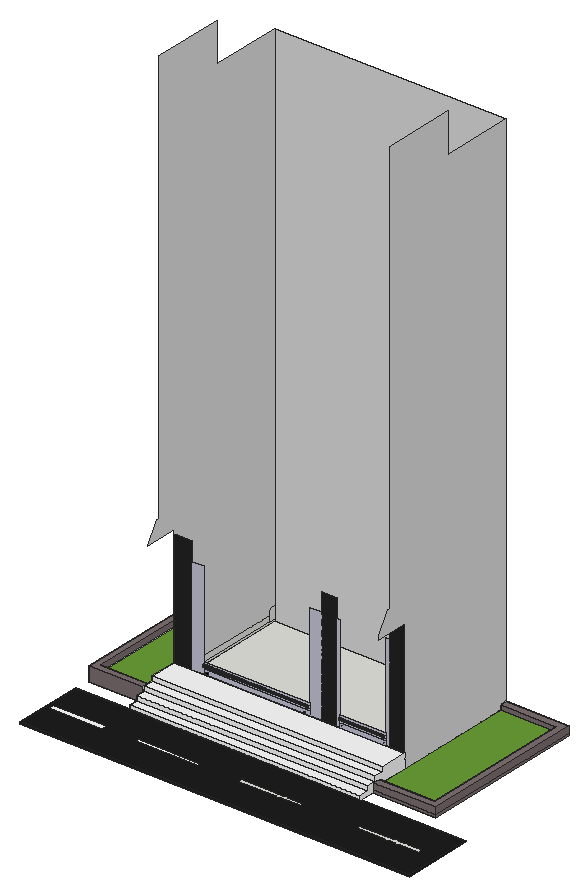
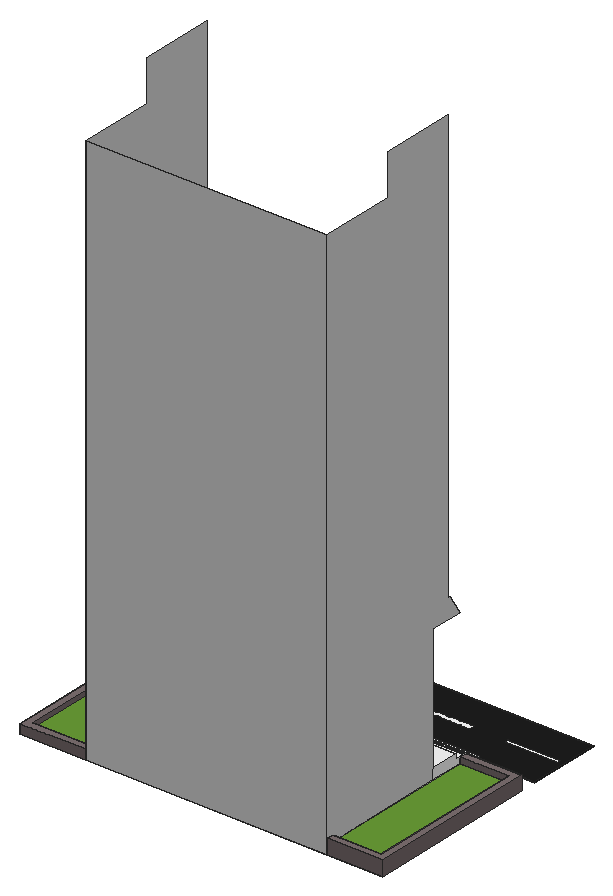
# SketchUp Ruby script. Lengths in millimetres.
U = 1.mm
M = Sketchup.active_model
def pt(a) = Geom::Point3d.new(a.map { |v| v * U })
def face(e, loops, mat)
  f = e.add_face(loops[0].map { |a| pt(a) })
  loops[1..].each { |l| e.add_face(l.map { |a| pt(a) }).erase! }
  f.material = f.back_material = mat if mat
  f
end
# faces: each face lists its corners as indices into pts; further lists are holes
def faces(e, pts, list, mat = nil) = list.each { |f| face(e, (f[0].is_a?(Array) ? f : [f]).map { |l| l.map { |i| pts[i] } }, mat) }
# xy, xz, yz: faces in a plane at the given z, y or x. An outline is a flat list of corners, or four numbers for a rectangle; further outlines are holes
def ring(l) = l.size == 4 ? [[l[0], l[1]], [l[2], l[1]], [l[2], l[3]], [l[0], l[3]]] : l.each_slice(2).to_a
def flat(e, list, mat, &to3) = list.each { |f| face(e, (f[0].is_a?(Array) ? f : [f]).map { |l| ring(l).map { |u, v| to3.(u, v) } }, mat) }
def xy(e, z, list, mat = nil) = flat(e, list, mat) { |x, y| [x, y, z] }
def xz(e, y, list, mat = nil) = flat(e, list, mat) { |x, z| [x, y, z] }
def yz(e, x, list, mat = nil) = flat(e, list, mat) { |y, z| [x, y, z] }
def lines(e, pts, list) = list.each { |a, b| e.add_line(pt(pts[a]), pt(pts[b])) }
# prism: a flat outline (further loops are holes) pulled along v
def prism(e, loops, v, mat = nil)
  f = face(e, loops, mat); d = Geom::Vector3d.new(v.map { |x| x * U })
  f.pushpull(f.normal.samedirection?(d) ? d.length : -d.length)
end
def box(e, o, s, mat = nil) = prism(e, [[o, [o[0] + s[0], o[1], o[2]], [o[0] + s[0], o[1] + s[1], o[2]], [o[0], o[1] + s[1], o[2]]]], [0, 0, s[2]], mat)
def at(x, y, z, deg = 0) = Geom::Transformation.translation(pt([x, y, z])) * Geom::Transformation.rotation(ORIGIN, Z_AXIS, deg.degrees)
def axes(o, x, y, z) = Geom::Transformation.new([*x, 0, *y, 0, *z, 0, *pt(o).to_a, 1])
def part(name) = M.definitions.add(name)
# library, detail: a bought-in or finely detailed component or shape, given as its bounding box
def library(name, o, s) = part(name).tap { |d| box(d.entities, o, s) }
def detail(e, o, s) = box(e.add_group.entities, o, s)
def put(e, d, t, mat = nil) = e.add_instance(d, t).tap { |i| i.material = mat if mat }
def group(e, t, mat = nil) = e.add_group.tap { |g| g.transformation = t; g.material = mat if mat }.entities
root = M.entities
M.materials.add("[0116_Lavender]").color = [197, 197, 214]
M.materials.add("[0128_White]1").color = [255, 255, 255]
M.materials.add("[0130_Gainsboro]").color = [220, 220, 220]
M.materials.add("[0136_Charcoal]").color = [35, 35, 35]
M.materials.add("[0137_Black]").color = [0, 0, 0]
M.materials.add("[Asphalt Stamped Brick]").color = [124, 111, 112]
M.materials.add("[Blacktop New]").color = [30, 30, 30]
M.materials.add("[Carrera Marble]").color = [252, 252, 252]
M.materials.add("[Grass Dark Green]").color = [106, 157, 55]
xy(root,-136.5,[[7076.1,9232.9,37556.1,16548.1],[0,11366.5,7076.1,33312.1],[37556.1,11366.5,45838.4,33312.1],[7076.1,16548.1,37556.1,33312.1]])
xy(root,-136.5,[[0,0,51467,9232.9]],"[Blacktop New]")
xy(root,15.9,[[25341.5,4311.6,33627.1,4921.2],[40973.6,4311.6,49259.3,4921.2]])
xy(root,15.9,[[553.8,4311.6,7431.8,4921.2],[11711.2,4311.6,19996.9,4921.2]],"[0128_White]1")
xy(root,15.9,[[[0,0,51467,9232.9],[40973.6,4311.6,49259.3,4921.2],[25341.5,4311.6,33627.1,4921.2],[11711.2,4311.6,19996.9,4921.2],[553.8,4311.6,7431.8,4921.2]]],"[Blacktop New]")
xy(root,168.3,[[914.4,12280.9,7076.1,32397.7]])
xy(root,473.1,[[7076.1,9232.9,37556.1,10452.1]],"[Carrera Marble]")
xy(root,473.1,[[37556.1,12280.9,44924,32397.7]],"[Grass Dark Green]")
xy(root,930.3,[[914.4,12280.9,7076.1,32397.7]],"[Grass Dark Green]")
xy(root,1082.7,[[37556.1,11366.5,45838.4,11366.5,45838.4,33312.1,37556.1,33312.1,37556.1,32397.7,44924,32397.7,44924,12280.9,37556.1,12280.9]],"[Asphalt Stamped Brick]")
xy(root,1082.7,[[7076.1,10452.1,37556.1,11671.3]],"[Carrera Marble]")
xy(root,1692.3,[[0,11366.5,7076.1,11366.5,7076.1,12280.9,914.4,12280.9,914.4,32397.7,7076.1,32397.7,7076.1,33312.1,0,33312.1]],"[Asphalt Stamped Brick]")
xy(root,1692.3,[[7076.1,11671.3,37556.1,12890.5]],"[Carrera Marble]")
xy(root,2301.9,[[7076.1,12890.5,37556.1,16548.1]],"[Carrera Marble]")
xz(root,0,[[0,-136.5,51467,15.9]],"[Blacktop New]")
xz(root,9232.9,[[0,-136.5,7076.1,15.9],[37556.1,-136.5,51467,15.9]],"[Blacktop New]")
xz(root,9232.9,[[7076.1,-136.5,37556.1,15.9],[7076.1,15.9,37556.1,473.1]],"[Carrera Marble]")
xz(root,10452.1,[[7076.1,473.1,37556.1,1082.7]],"[Carrera Marble]")
xz(root,11366.5,[[0,-136.5,7076.1,1692.3],[37556.1,-136.5,45838.4,168.3],[37556.1,168.3,45838.4,1082.7]],"[Asphalt Stamped Brick]")
xz(root,11671.3,[[7076.1,1082.7,37556.1,1692.3]],"[Carrera Marble]")
xz(root,12280.9,[[914.4,168.3,7076.1,930.3],[37556.1,473.1,44924,1082.7]])
xz(root,12280.9,[[914.4,930.3,7076.1,1692.3]],"[Asphalt Stamped Brick]")
xz(root,12890.5,[[7076.1,1692.3,37556.1,2301.9]],"[Carrera Marble]")
xz(root,16548.1,[[7076.1,-136.5,37556.1,473.1],[7076.1,473.1,37556.1,1082.7],[7076.1,1082.7,37556.1,1692.3],[7076.1,1692.3,37556.1,2301.9],[11038.5,3216.3,25059.3,3521.1],
  [29021.7,3216.3,35117.7,3521.1]])
xz(root,16548.1,[[9514.5,2301.9,11038.5,15103.5],[[11038.5,2301.9,25059.3,2911.5],[24427,2390.4,24399.4,2396.3,24373.6,2407.8,24350.8,2424.3,24331.9,2445.3,24317.8,2469.7,24309.1,2496.6,24306.2,2524.6,24309.1,2552.7,24317.8,2579.5,24331.9,2603.9,24350.8,2624.9,24373.6,2641.5,24399.4,2653,24427,2658.8,24455.2,2658.8,24482.8,2653,24508.6,2641.5,24531.4,2624.9,24550.3,2603.9,24564.4,2579.5,24573.1,2552.7,24576,2524.6,24573.1,2496.6,24564.4,2469.7,24550.3,2445.3,24531.4,2424.3,24508.6,2407.8,24482.8,2396.3,24455.2,2390.4],[11495.2,2390.4,11467.6,2396.3,11441.9,2407.8,11419,2424.3,11400.2,2445.3,11386.1,2469.7,11377.3,2496.6,11374.4,2524.6,11377.3,2552.7,11386.1,2579.5,11400.2,2603.9,11419,2624.9,11441.9,2641.5,11467.6,2653,11495.2,2658.8,11523.4,2658.8,11551,2653,11576.8,2641.5,11599.6,2624.9,11618.5,2603.9,11632.6,2579.5,11641.3,2552.7,11644.3,2524.6,11641.3,2496.6,11632.6,2469.7,11618.5,2445.3,11599.6,2424.3,11576.8,2407.8,11551,2396.3,11523.4,2390.4]],[25059.3,2301.9,26583.3,15103.5],[28564.5,2301.9,29021.7,15103.5],[[29021.7,2301.9,35117.7,2911.5],[34872.3,2572,34893,2673.6],[29327.2,2572,29347.8,2673.6]],
  [35117.7,2301.9,35574.9,15103.5],[11038.5,2911.5,25059.3,3216.3],[29021.7,2911.5,35117.7,3216.3],[11038.5,3521.1,25059.3,3825.9],[29021.7,3521.1,35117.7,3825.9]],"[0116_Lavender]")
xz(root,16548.1,[[7076.1,2301.9,9514.5,17541.9],[26583.3,2301.9,28564.5,17541.9],[35574.9,2301.9,37556.1,17541.9]],"[0136_Charcoal]")
xz(root,16548.1,[[11495.2,2390.4,11523.4,2390.4,11551,2396.3,11576.8,2407.8,11599.6,2424.3,11618.5,2445.3,11632.6,2469.7,11641.3,2496.6,11644.3,2524.6,11641.3,2552.7,11632.6,2579.5,11618.5,2603.9,11599.6,2624.9,11576.8,2641.5,11551,2653,11523.4,2658.8,11495.2,2658.8,11467.6,2653,11441.9,2641.5,11419,2624.9,11400.2,2603.9,11386.1,2579.5,11377.3,2552.7,11374.4,2524.6,11377.3,2496.6,11386.1,2469.7,11400.2,2445.3,11419,2424.3,11441.9,2407.8,11467.6,2396.3],[24427,2390.4,24455.2,2390.4,24482.8,2396.3,24508.6,2407.8,24531.4,2424.3,24550.3,2445.3,24564.4,2469.7,24573.1,2496.6,24576,2524.6,24573.1,2552.7,24564.4,2579.5,24550.3,2603.9,24531.4,2624.9,24508.6,2641.5,24482.8,2653,24455.2,2658.8,24427,2658.8,24399.4,2653,24373.6,2641.5,24350.8,2624.9,24331.9,2603.9,24317.8,2579.5,24309.1,2552.7,24306.2,2524.6,24309.1,2496.6,24317.8,2469.7,24331.9,2445.3,24350.8,2424.3,24373.6,2407.8,24399.4,2396.3],[29327.2,2572,29347.8,2673.6],[34872.3,2572,34893,2673.6]],"[0137_Black]")
xz(root,32397.7,[[914.4,168.3,7076.1,930.3]])
xz(root,32397.7,[[37556.1,473.1,44924,1082.7],[914.4,930.3,7076.1,1692.3]],"[Asphalt Stamped Brick]")
xz(root,33312.1,[[7076.1,-136.5,37556.1,69967.5]],"[0130_Gainsboro]")
xz(root,33312.1,[[0,-136.5,7076.1,1692.3],[37556.1,-136.5,45838.4,1082.7]],"[Asphalt Stamped Brick]")
yz(root,0,[[11366.5,-136.5,33312.1,1692.3]],"[Asphalt Stamped Brick]")
yz(root,0,[[0,-136.5,9232.9,15.9]],"[Blacktop New]")
yz(root,914.4,[[12280.9,168.3,32397.7,930.3]])
yz(root,914.4,[[12280.9,930.3,32397.7,1692.3]],"[Asphalt Stamped Brick]")
yz(root,7076.1,[[11366.5,-136.5,16548.1,168.3],[16548.1,-136.5,33312.1,168.3],[12280.9,168.3,16548.1,930.3],[16548.1,168.3,32397.7,930.3],[32397.7,168.3,33312.1,1692.3],
  [11366.5,1082.7,11671.3,1692.3]])
yz(root,7076.1,[[16548.1,930.3,16548.1,17999.1,12280.9,17999.1,13804.9,20437.5,14109.7,20437.5,14109.7,75149.1,23710.9,75149.1,23710.9,69967.5,33312.1,69967.5,33312.1,1692.3,32397.7,1692.3,32397.7,930.3]],"[0130_Gainsboro]")
yz(root,7076.1,[[9232.9,-136.5,9232.9,473.1,10452.1,473.1,10452.1,1082.7,11366.5,1082.7,11366.5,-136.5],[11366.5,168.3,11366.5,1082.7,11671.3,1082.7,11671.3,1692.3,12280.9,1692.3,12280.9,168.3],[12280.9,930.3,12280.9,1692.3,12890.5,1692.3,12890.5,2301.9,16548.1,2301.9,16548.1,930.3]],"[Carrera Marble]")
yz(root,11038.5,[[16548.1,3216.3,16536.2,3221.6,16524.8,3227.9,16514,3235,16503.7,3243,16494.1,3251.8,16485.2,3261.3,16477.1,3271.4,16469.8,3282.2,16463.4,3293.5,16458,3305.3,16453.4,3317.5,16449.9,3330,16447.3,3342.8,16445.8,3355.7,16445.3,3368.7,16445.8,3381.7,16447.3,3394.6,16449.9,3407.3,16453.4,3419.8,16458,3432,16463.4,3443.8,16469.8,3455.1,16477.1,3465.9,16485.2,3476.1,16494.1,3485.6,16503.7,3494.4,16514,3502.3,16524.8,3509.5,16536.2,3515.7,16548.1,3521.1]])
yz(root,25059.3,[[16548.1,3216.3,16548.1,3521.1,16536.2,3515.7,16524.8,3509.5,16514,3502.3,16503.7,3494.4,16494.1,3485.6,16485.2,3476.1,16477.1,3465.9,16469.8,3455.1,16463.4,3443.8,16458,3432,16453.4,3419.8,16449.9,3407.3,16447.3,3394.6,16445.8,3381.7,16445.3,3368.7,16445.8,3355.7,16447.3,3342.8,16449.9,3330,16453.4,3317.5,16458,3305.3,16463.4,3293.5,16469.8,3282.2,16477.1,3271.4,16485.2,3261.3,16494.1,3251.8,16503.7,3243,16514,3235,16524.8,3227.9,16536.2,3221.6]])
yz(root,29021.7,[[16548.1,3216.3,16540.1,3216.5,16532.2,3217.1,16524.3,3218.2,16516.4,3219.6,16508.7,3221.5,16501,3223.7,16493.5,3226.4,16486.1,3229.5,16478.9,3232.9,16471.9,3236.7,16465.1,3240.9,16458.5,3245.4,16452.2,3250.2,16446.1,3255.4,16440.3,3260.9,16434.8,3266.7,16429.7,3272.8,16424.8,3279.1,16420.3,3285.7,16416.1,3292.5,16412.3,3299.5,16408.9,3306.7,16405.8,3314.1,16403.2,3321.6,16400.9,3329.2,16399,3337,16397.6,3344.8,16396.5,3352.7,16395.9,3360.7,16395.7,3368.7,16395.9,3376.7,16396.5,3384.6,16397.6,3392.5,16399,3400.4,16400.9,3408.1,16403.2,3415.8,16405.8,3423.3,16408.9,3430.7,16412.3,3437.9,16416.1,3444.9,16420.3,3451.7,16424.8,3458.3,16429.7,3464.6,16434.8,3470.7,16440.3,3476.4,16446.1,3481.9,16452.2,3487.1,16458.5,3492,16465.1,3496.5,16471.9,3500.7,16478.9,3504.5,16486.1,3507.9,16493.5,3511,16501,3513.6,16508.7,3515.9,16516.4,3517.7,16524.3,3519.2,16532.2,3520.2,16540.1,3520.9,16548.1,3521.1]])
yz(root,35117.7,[[16548.1,3216.3,16548.1,3521.1,16540.1,3520.9,16532.2,3520.2,16524.3,3519.2,16516.4,3517.7,16508.7,3515.9,16501,3513.6,16493.5,3511,16486.1,3507.9,16478.9,3504.5,16471.9,3500.7,16465.1,3496.5,16458.5,3492,16452.2,3487.1,16446.1,3481.9,16440.3,3476.4,16434.8,3470.7,16429.7,3464.6,16424.8,3458.3,16420.3,3451.7,16416.1,3444.9,16412.3,3437.9,16408.9,3430.7,16405.8,3423.3,16403.2,3415.8,16400.9,3408.1,16399,3400.4,16397.6,3392.5,16396.5,3384.6,16395.9,3376.7,16395.7,3368.7,16395.9,3360.7,16396.5,3352.7,16397.6,3344.8,16399,3337,16400.9,3329.2,16403.2,3321.6,16405.8,3314.1,16408.9,3306.7,16412.3,3299.5,16416.1,3292.5,16420.3,3285.7,16424.8,3279.1,16429.7,3272.8,16434.8,3266.7,16440.3,3260.9,16446.1,3255.4,16452.2,3250.2,16458.5,3245.4,16465.1,3240.9,16471.9,3236.7,16478.9,3232.9,16486.1,3229.5,16493.5,3226.4,16501,3223.7,16508.7,3221.5,16516.4,3219.6,16524.3,3218.2,16532.2,3217.1,16540.1,3216.5]])
yz(root,37556.1,[[11366.5,-136.5,16548.1,-136.5,16548.1,473.1,12280.9,473.1,12280.9,168.3,11366.5,168.3],[16548.1,-136.5,33312.1,-136.5,33312.1,168.3,32397.7,168.3,32397.7,473.1,16548.1,473.1],[32397.7,168.3,33312.1,1082.7]])
yz(root,37556.1,[[16548.1,473.1,32397.7,473.1,32397.7,1082.7,33312.1,1082.7,33312.1,69967.5,23710.9,69967.5,23710.9,75149.1,14109.7,75149.1,14109.7,20437.5,13804.9,20437.5,12280.9,17999.1,12280.9,17541.9,16548.1,17541.9]],"[0130_Gainsboro]")
yz(root,37556.1,[[9232.9,-136.5,11366.5,-136.5,11366.5,1082.7,10452.1,1082.7,10452.1,473.1,9232.9,473.1],[11366.5,168.3,12280.9,1082.7],[12280.9,473.1,16548.1,473.1,16548.1,2301.9,12890.5,2301.9,12890.5,1692.3,11671.3,1692.3,11671.3,1082.7,12280.9,1082.7]],"[Carrera Marble]")
yz(root,44924,[[12280.9,473.1,32397.7,1082.7]],"[Asphalt Stamped Brick]")
yz(root,45838.4,[[11366.5,-136.5,33312.1,168.3],[11366.5,168.3,33312.1,1082.7]],"[Asphalt Stamped Brick]")
yz(root,51467,[[0,-136.5,9232.9,15.9]],"[Blacktop New]")
p = [[25059.3,16548.1,3216.3],[25059.3,16536.2,3221.6],[11038.5,16536.2,3221.6],[11038.5,16548.1,3216.3],[35117.7,16548.1,3216.3],[35117.7,16540.1,3216.5],
  [29021.7,16540.1,3216.5],[29021.7,16548.1,3216.3],[35117.7,16532.2,3217.1],[29021.7,16532.2,3217.1],[35117.7,16524.3,3218.2],[29021.7,16524.3,3218.2],
  [35117.7,16516.4,3219.6],[29021.7,16516.4,3219.6],[35117.7,16508.7,3221.5],[29021.7,16508.7,3221.5],[35117.7,16501,3223.7],[29021.7,16501,3223.7],
  [25059.3,16524.8,3227.9],[11038.5,16524.8,3227.9],[35117.7,16493.5,3226.4],[29021.7,16493.5,3226.4],[35117.7,16486.1,3229.5],[29021.7,16486.1,3229.5],
  [25059.3,16514,3235],[11038.5,16514,3235],[35117.7,16478.9,3232.9],[29021.7,16478.9,3232.9],[35117.7,16471.9,3236.7],[29021.7,16471.9,3236.7],
  [25059.3,16503.7,3243],[11038.5,16503.7,3243],[35117.7,16465.1,3240.9],[29021.7,16465.1,3240.9],[35117.7,16458.5,3245.4],[29021.7,16458.5,3245.4],
  [25059.3,16494.1,3251.8],[11038.5,16494.1,3251.8],[35117.7,16452.2,3250.2],[29021.7,16452.2,3250.2],[35117.7,16446.1,3255.4],[29021.7,16446.1,3255.4],
  [25059.3,16485.2,3261.3],[11038.5,16485.2,3261.3],[35117.7,16440.3,3260.9],[29021.7,16440.3,3260.9],[35117.7,16434.8,3266.7],[29021.7,16434.8,3266.7],
  [25059.3,16477.1,3271.4],[11038.5,16477.1,3271.4],[35117.7,16429.7,3272.8],[29021.7,16429.7,3272.8],[25059.3,16469.8,3282.2],[11038.5,16469.8,3282.2],
  [35117.7,16424.8,3279.1],[29021.7,16424.8,3279.1],[35117.7,16420.3,3285.7],[29021.7,16420.3,3285.7],[25059.3,16463.4,3293.5],[11038.5,16463.4,3293.5],
  [35117.7,16416.1,3292.5],[29021.7,16416.1,3292.5],[35117.7,16412.3,3299.5],[29021.7,16412.3,3299.5],[25059.3,16458,3305.3],[11038.5,16458,3305.3],
  [35117.7,16408.9,3306.7],[29021.7,16408.9,3306.7],[25059.3,16453.4,3317.5],[11038.5,16453.4,3317.5],[35117.7,16405.8,3314.1],[29021.7,16405.8,3314.1],
  [35117.7,16403.2,3321.6],[29021.7,16403.2,3321.6],[25059.3,16449.9,3330],[11038.5,16449.9,3330],[35117.7,16400.9,3329.2],[29021.7,16400.9,3329.2],
  [35117.7,16399,3337],[29021.7,16399,3337],[25059.3,16447.3,3342.8],[11038.5,16447.3,3342.8],[35117.7,16397.6,3344.8],[29021.7,16397.6,3344.8],
  [25059.3,16445.8,3355.7],[11038.5,16445.8,3355.7],[35117.7,16396.5,3352.7],[29021.7,16396.5,3352.7],[35117.7,16395.9,3360.7],[29021.7,16395.9,3360.7],
  [25059.3,16445.3,3368.7],[11038.5,16445.3,3368.7],[35117.7,16395.7,3368.7],[29021.7,16395.7,3368.7],[35117.7,16395.9,3376.7],[29021.7,16395.9,3376.7],
  [25059.3,16445.8,3381.7],[11038.5,16445.8,3381.7],[35117.7,16396.5,3384.6],[29021.7,16396.5,3384.6],[25059.3,16447.3,3394.6],[11038.5,16447.3,3394.6],
  [35117.7,16397.6,3392.5],[29021.7,16397.6,3392.5],[35117.7,16399,3400.4],[29021.7,16399,3400.4],[25059.3,16449.9,3407.3],[11038.5,16449.9,3407.3],
  [35117.7,16400.9,3408.1],[29021.7,16400.9,3408.1],[25059.3,16453.4,3419.8],[11038.5,16453.4,3419.8],[35117.7,16403.2,3415.8],[29021.7,16403.2,3415.8],
  [35117.7,16405.8,3423.3],[29021.7,16405.8,3423.3],[25059.3,16458,3432],[11038.5,16458,3432],[35117.7,16408.9,3430.7],[29021.7,16408.9,3430.7],
  [35117.7,16412.3,3437.9],[29021.7,16412.3,3437.9],[25059.3,16463.4,3443.8],[11038.5,16463.4,3443.8],[35117.7,16416.1,3444.9],[29021.7,16416.1,3444.9],
  [25059.3,16469.8,3455.1],[11038.5,16469.8,3455.1],[35117.7,16420.3,3451.7],[29021.7,16420.3,3451.7],[35117.7,16424.8,3458.3],[29021.7,16424.8,3458.3],
  [25059.3,16477.1,3465.9],[11038.5,16477.1,3465.9],[35117.7,16429.7,3464.6],[29021.7,16429.7,3464.6],[35117.7,16434.8,3470.7],[29021.7,16434.8,3470.7],
  [25059.3,16485.2,3476.1],[11038.5,16485.2,3476.1],[35117.7,16440.3,3476.4],[29021.7,16440.3,3476.4],[25059.3,16494.1,3485.6],[11038.5,16494.1,3485.6],
  [35117.7,16446.1,3481.9],[29021.7,16446.1,3481.9],[35117.7,16452.2,3487.1],[29021.7,16452.2,3487.1],[25059.3,16503.7,3494.4],[11038.5,16503.7,3494.4],
  [35117.7,16458.5,3492],[29021.7,16458.5,3492],[35117.7,16465.1,3496.5],[29021.7,16465.1,3496.5],[25059.3,16514,3502.3],[11038.5,16514,3502.3],
  [35117.7,16471.9,3500.7],[29021.7,16471.9,3500.7],[35117.7,16478.9,3504.5],[29021.7,16478.9,3504.5],[25059.3,16524.8,3509.5],[11038.5,16524.8,3509.5],
  [35117.7,16486.1,3507.9],[29021.7,16486.1,3507.9],[35117.7,16493.5,3511],[29021.7,16493.5,3511],[25059.3,16536.2,3515.7],[11038.5,16536.2,3515.7],
  [35117.7,16501,3513.6],[29021.7,16501,3513.6],[35117.7,16508.7,3515.9],[29021.7,16508.7,3515.9],[25059.3,16548.1,3521.1],[11038.5,16548.1,3521.1],
  [35117.7,16516.4,3517.7],[29021.7,16516.4,3517.7],[35117.7,16524.3,3519.2],[29021.7,16524.3,3519.2],[35117.7,16532.2,3520.2],[29021.7,16532.2,3520.2],
  [35117.7,16540.1,3520.9],[29021.7,16540.1,3520.9],[35117.7,16548.1,3521.1],[29021.7,16548.1,3521.1]]
faces(root,p,[[0,1,2,3],[4,5,6,7],[5,8,9,6],[8,10,11,9],[10,12,13,11],[12,14,15,13],[14,16,17,15],[1,18,19,2],
  [16,20,21,17],[20,22,23,21],[18,24,25,19],[22,26,27,23],[26,28,29,27],[24,30,31,25],[28,32,33,29],[32,34,35,33],
  [30,36,37,31],[34,38,39,35],[38,40,41,39],[36,42,43,37],[40,44,45,41],[44,46,47,45],[42,48,49,43],[46,50,51,47],
  [48,52,53,49],[50,54,55,51],[54,56,57,55],[52,58,59,53],[56,60,61,57],[60,62,63,61],[58,64,65,59],[62,66,67,63],
  [64,68,69,65],[66,70,71,67],[70,72,73,71],[68,74,75,69],[72,76,77,73],[76,78,79,77],[74,80,81,75],[78,82,83,79],
  [80,84,85,81],[82,86,87,83],[86,88,89,87],[84,90,91,85],[88,92,93,89],[92,94,95,93],[90,96,97,91],[94,98,99,95],
  [96,100,101,97],[98,102,103,99],[102,104,105,103],[100,106,107,101],[104,108,109,105],[106,110,111,107],[108,112,113,109],[112,114,115,113],
  [110,116,117,111],[114,118,119,115],[118,120,121,119],[116,122,123,117],[120,124,125,121],[122,126,127,123],[124,128,129,125],[128,130,131,129],
  [126,132,133,127],[130,134,135,131],[134,136,137,135],[132,138,139,133],[136,140,141,137],[138,142,143,139],[140,144,145,141],[144,146,147,145],
  [142,148,149,143],[146,150,151,147],[150,152,153,151],[148,154,155,149],[152,156,157,153],[156,158,159,157],[154,160,161,155],[158,162,163,159],
  [162,164,165,163],[160,166,167,161],[164,168,169,165],[168,170,171,169],[166,172,173,167],[170,174,175,171],[174,176,177,175],[176,178,179,177],
  [178,180,181,179],[180,182,183,181]],"[0116_Lavender]")
